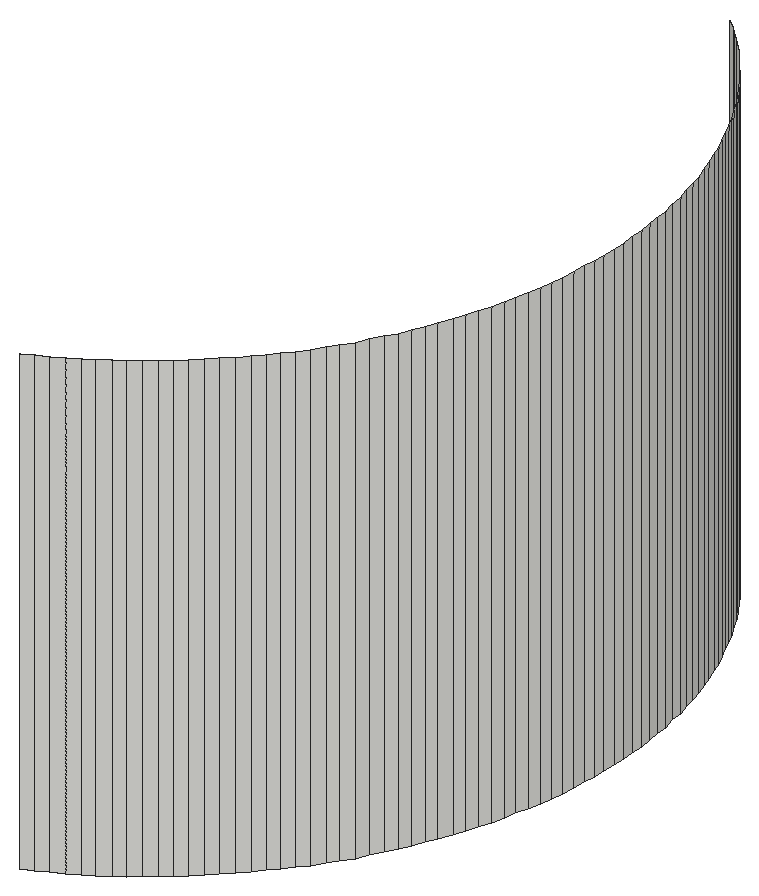
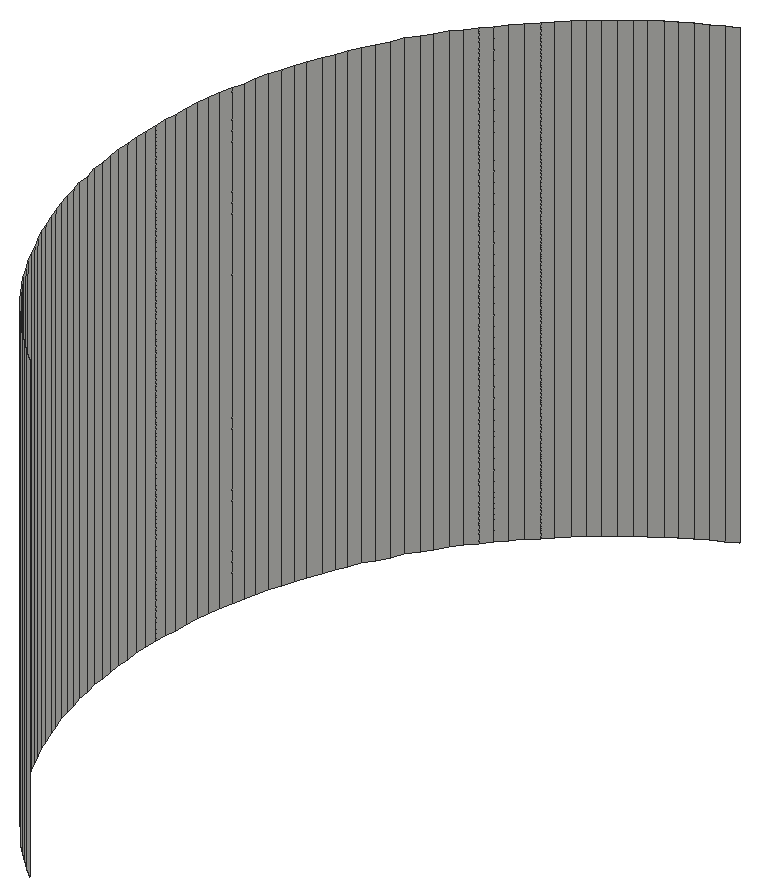
# SketchUp Ruby script. Lengths in inches.
U = 1.inch
M = Sketchup.active_model
def pt(a) = Geom::Point3d.new(a.map { |v| v * U })
def face(e, loops, mat)
  f = e.add_face(loops[0].map { |a| pt(a) })
  loops[1..].each { |l| e.add_face(l.map { |a| pt(a) }).erase! }
  f.material = f.back_material = mat if mat
  f
end
# faces: each face lists its corners as indices into pts; further lists are holes
def faces(e, pts, list, mat = nil) = list.each { |f| face(e, (f[0].is_a?(Array) ? f : [f]).map { |l| l.map { |i| pts[i] } }, mat) }
# xy, xz, yz: faces in a plane at the given z, y or x. An outline is a flat list of corners, or four numbers for a rectangle; further outlines are holes
def ring(l) = l.size == 4 ? [[l[0], l[1]], [l[2], l[1]], [l[2], l[3]], [l[0], l[3]]] : l.each_slice(2).to_a
def flat(e, list, mat, &to3) = list.each { |f| face(e, (f[0].is_a?(Array) ? f : [f]).map { |l| ring(l).map { |u, v| to3.(u, v) } }, mat) }
def xy(e, z, list, mat = nil) = flat(e, list, mat) { |x, y| [x, y, z] }
def xz(e, y, list, mat = nil) = flat(e, list, mat) { |x, z| [x, y, z] }
def yz(e, x, list, mat = nil) = flat(e, list, mat) { |y, z| [x, y, z] }
def lines(e, pts, list) = list.each { |a, b| e.add_line(pt(pts[a]), pt(pts[b])) }
# prism: a flat outline (further loops are holes) pulled along v
def prism(e, loops, v, mat = nil)
  f = face(e, loops, mat); d = Geom::Vector3d.new(v.map { |x| x * U })
  f.pushpull(f.normal.samedirection?(d) ? d.length : -d.length)
end
def box(e, o, s, mat = nil) = prism(e, [[o, [o[0] + s[0], o[1], o[2]], [o[0] + s[0], o[1] + s[1], o[2]], [o[0], o[1] + s[1], o[2]]]], [0, 0, s[2]], mat)
def at(x, y, z, deg = 0) = Geom::Transformation.translation(pt([x, y, z])) * Geom::Transformation.rotation(ORIGIN, Z_AXIS, deg.degrees)
def axes(o, x, y, z) = Geom::Transformation.new([*x, 0, *y, 0, *z, 0, *pt(o).to_a, 1])
def part(name) = M.definitions.add(name)
# library, detail: a bought-in or finely detailed component or shape, given as its bounding box
def library(name, o, s) = part(name).tap { |d| box(d.entities, o, s) }
def detail(e, o, s) = box(e.add_group.entities, o, s)
def put(e, d, t, mat = nil) = e.add_instance(d, t).tap { |i| i.material = mat if mat }
def group(e, t, mat = nil) = e.add_group.tap { |g| g.transformation = t; g.material = mat if mat }.entities
root = M.entities
yz(root,217.39,[[319.72,231,319.8,234],[320.19,231,320.27,234]])
yz(root,217.4,[[319.875,231,319.95,234],[319.95,231,320.03,234],[320.03,231,320.11,234]])
p = [[215.79,317.34,231],[215.72,317.31,231],[215.72,317.31,234],[215.79,317.34,234],[215.86,317.38,231],[215.86,317.38,234],
  [216,317.46,231],[215.93,317.42,231],[215.93,317.42,234],[216,317.46,234],[216.0625,317.5,231],[216.0625,317.5,234],
  [216.19,317.59,231],[216.125,317.55,231],[216.125,317.55,234],[216.19,317.59,234],[216.25,317.64,231],[216.25,317.64,234],
  [216.3125,317.69,231],[216.3125,317.69,234],[216.375,317.74,231],[216.375,317.74,234],[216.43,317.79,231],[216.43,317.79,234],
  [216.49,317.85,231],[216.49,317.85,234],[216.54,317.9,231],[216.54,317.9,234],[216.6,317.96,231],[216.6,317.96,234],
  [216.65,318.02,231],[216.65,318.02,234],[216.7,318.08,231],[216.7,318.08,234],[216.75,318.14,231],[216.75,318.14,234],
  [216.8,318.2,231],[216.8,318.2,234],[216.85,318.26,231],[216.85,318.26,234],[216.89,318.33,231],[216.89,318.33,234],
  [216.93,318.39,231],[216.93,318.39,234],[216.98,318.46,231],[216.98,318.46,234],[217.05,318.6,231],[217.01,318.53,231],
  [217.01,318.53,234],[217.05,318.6,234],[217.09,318.67,231],[217.09,318.67,234],[217.15,318.81,231],[217.12,318.74,231],
  [217.12,318.74,234],[217.15,318.81,234],[217.18,318.88,231],[217.18,318.88,234],[217.21,318.96,231],[217.21,318.96,234],
  [217.26,319.1,231],[217.24,319.03,231],[217.24,319.03,234],[217.26,319.1,234],[217.29,319.18,231],[217.29,319.18,234],
  [217.31,319.26,231],[217.31,319.26,234],[217.34,319.41,231],[217.32,319.33,231],[217.32,319.33,234],[217.34,319.41,234],
  [217.36,319.49,231],[217.36,319.49,234],[217.37,319.5625,231],[217.37,319.5625,234],[217.39,319.72,231],[217.38,319.64,231],
  [217.38,319.64,234],[217.39,319.72,234],[217.4,319.875,231],[217.39,319.8,231],[217.39,319.8,234],[217.4,319.875,234],
  [217.39,320.19,231],[217.4,320.11,231],[217.4,320.11,234],[217.39,320.19,234],[217.37,320.42,231],[217.38,320.35,231],
  [217.38,320.35,234],[217.37,320.42,234],[217.39,320.27,231],[217.39,320.27,234],[217.36,320.5,231],[217.36,320.5,234],
  [217.34,320.58,231],[217.34,320.58,234],[217.33,320.66,231],[217.33,320.66,234],[217.29,320.81,231],[217.31,320.73,231],
  [217.31,320.73,234],[217.29,320.81,234],[217.27,320.88,231],[217.27,320.88,234],[217.24,320.96,231],[217.24,320.96,234],
  [217.1875,321.11,231],[217.22,321.03,231],[217.22,321.03,234],[217.1875,321.11,234],[217.16,321.18,231],[217.16,321.18,234],
  [217.125,321.25,231],[217.125,321.25,234],[217.06,321.39,231],[217.09,321.32,231],[217.09,321.32,234],[217.06,321.39,234],
  [217.02,321.46,231],[217.02,321.46,234],[216.94,321.6,231],[216.98,321.53,231],[216.98,321.53,234],[216.94,321.6,234],
  [216.9,321.66,231],[216.9,321.66,234],[216.81,321.79,231],[216.85,321.73,231],[216.85,321.73,234],[216.81,321.79,234],
  [216.76,321.85,231],[216.76,321.85,234],[216.66,321.97,231],[216.71,321.91,231],[216.71,321.91,234],[216.66,321.97,234],
  [216.55,322.09,231],[216.61,322.03,231],[216.61,322.03,234],[216.55,322.09,234],[216.44,322.2,231],[216.5,322.14,231],
  [216.5,322.14,234],[216.44,322.2,234],[216.38,322.25,231],[216.38,322.25,234]]
faces(root,p,[[0,1,2,3],[4,0,3,5],[6,7,8,9],[7,4,5,8],[10,6,9,11],[12,13,14,15],[13,10,11,14],[16,12,15,17],
  [18,16,17,19],[20,18,19,21],[22,20,21,23],[24,22,23,25],[26,24,25,27],[28,26,27,29],[30,28,29,31],[32,30,31,33],
  [34,32,33,35],[36,34,35,37],[38,36,37,39],[40,38,39,41],[42,40,41,43],[44,42,43,45],[46,47,48,49],[47,44,45,48],
  [50,46,49,51],[52,53,54,55],[53,50,51,54],[56,52,55,57],[58,56,57,59],[60,61,62,63],[61,58,59,62],[64,60,63,65],
  [66,64,65,67],[68,69,70,71],[69,66,67,70],[72,68,71,73],[74,72,73,75],[76,77,78,79],[77,74,75,78],[80,81,82,83],
  [84,85,86,87],[88,89,90,91],[89,92,93,90],[94,88,91,95],[96,94,95,97],[98,96,97,99],[100,101,102,103],[101,98,99,102],
  [104,100,103,105],[106,104,105,107],[108,109,110,111],[109,106,107,110],[112,108,111,113],[114,112,113,115],[116,117,118,119],[117,114,115,118],
  [120,116,119,121],[122,123,124,125],[123,120,121,124],[126,122,125,127],[128,129,130,131],[129,126,127,130],[132,128,131,133],[134,135,136,137],
  [135,132,133,136],[138,139,140,141],[139,134,137,140],[142,143,144,145],[143,138,141,144],[146,142,145,147]])
